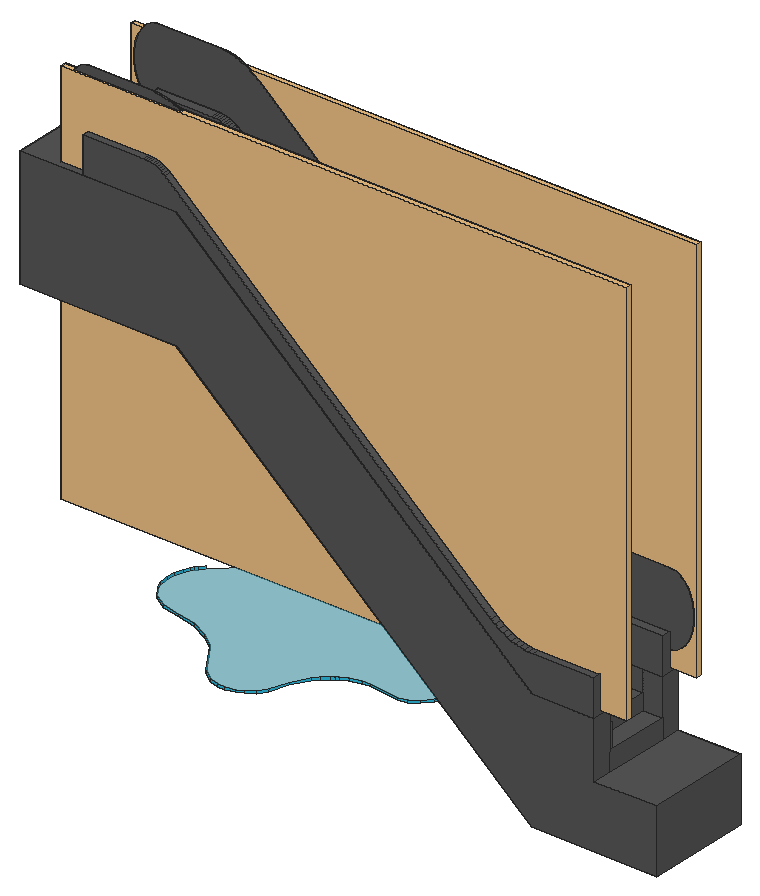
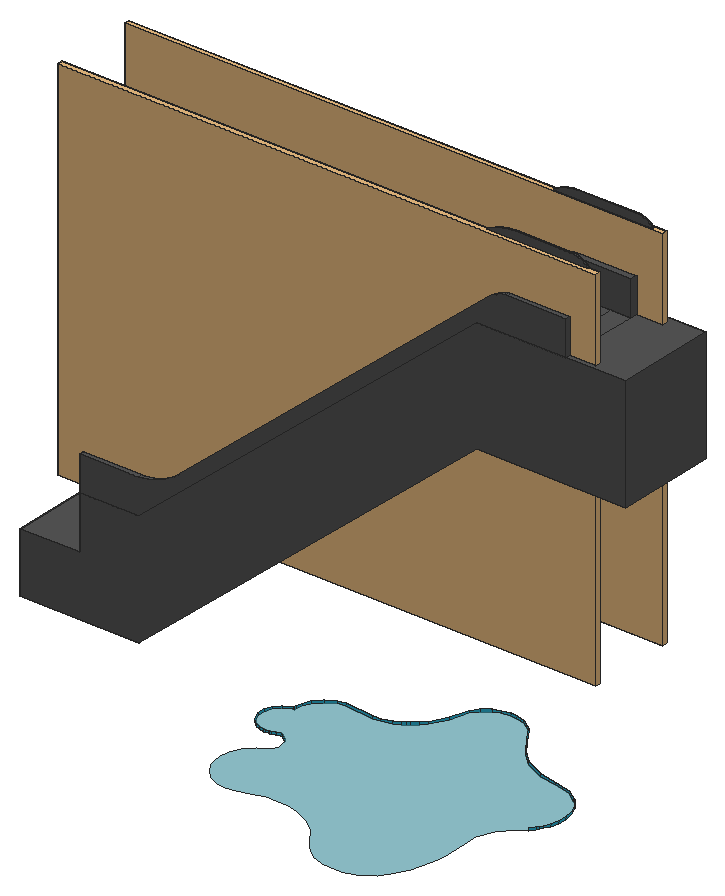
# SketchUp Ruby script. Lengths in inches.
U = 1.inch
M = Sketchup.active_model
def pt(a) = Geom::Point3d.new(a.map { |v| v * U })
def face(e, loops, mat)
  f = e.add_face(loops[0].map { |a| pt(a) })
  loops[1..].each { |l| e.add_face(l.map { |a| pt(a) }).erase! }
  f.material = f.back_material = mat if mat
  f
end
# faces: each face lists its corners as indices into pts; further lists are holes
def faces(e, pts, list, mat = nil) = list.each { |f| face(e, (f[0].is_a?(Array) ? f : [f]).map { |l| l.map { |i| pts[i] } }, mat) }
# xy, xz, yz: faces in a plane at the given z, y or x. An outline is a flat list of corners, or four numbers for a rectangle; further outlines are holes
def ring(l) = l.size == 4 ? [[l[0], l[1]], [l[2], l[1]], [l[2], l[3]], [l[0], l[3]]] : l.each_slice(2).to_a
def flat(e, list, mat, &to3) = list.each { |f| face(e, (f[0].is_a?(Array) ? f : [f]).map { |l| ring(l).map { |u, v| to3.(u, v) } }, mat) }
def xy(e, z, list, mat = nil) = flat(e, list, mat) { |x, y| [x, y, z] }
def xz(e, y, list, mat = nil) = flat(e, list, mat) { |x, z| [x, y, z] }
def yz(e, x, list, mat = nil) = flat(e, list, mat) { |y, z| [x, y, z] }
def lines(e, pts, list) = list.each { |a, b| e.add_line(pt(pts[a]), pt(pts[b])) }
# prism: a flat outline (further loops are holes) pulled along v
def prism(e, loops, v, mat = nil)
  f = face(e, loops, mat); d = Geom::Vector3d.new(v.map { |x| x * U })
  f.pushpull(f.normal.samedirection?(d) ? d.length : -d.length)
end
def box(e, o, s, mat = nil) = prism(e, [[o, [o[0] + s[0], o[1], o[2]], [o[0] + s[0], o[1] + s[1], o[2]], [o[0], o[1] + s[1], o[2]]]], [0, 0, s[2]], mat)
def at(x, y, z, deg = 0) = Geom::Transformation.translation(pt([x, y, z])) * Geom::Transformation.rotation(ORIGIN, Z_AXIS, deg.degrees)
def axes(o, x, y, z) = Geom::Transformation.new([*x, 0, *y, 0, *z, 0, *pt(o).to_a, 1])
def part(name) = M.definitions.add(name)
# library, detail: a bought-in or finely detailed component or shape, given as its bounding box
def library(name, o, s) = part(name).tap { |d| box(d.entities, o, s) }
def detail(e, o, s) = box(e.add_group.entities, o, s)
def put(e, d, t, mat = nil) = e.add_instance(d, t).tap { |i| i.material = mat if mat }
def group(e, t, mat = nil) = e.add_group.tap { |g| g.transformation = t; g.material = mat if mat }.entities
root = M.entities
M.materials.add("[Color M06]").color = [86, 86, 86]
M.materials.add("[Water Pool Light]").color = [62, 149, 166]
M.materials["[Water Pool Light]"].alpha = 0.6
M.materials.add("[Water Sparkling]").color = [45, 182, 216]
c1 = library("Group9\#2",[-51.57,-27.17,6.46],[325.75,3.15,149.29])
c2 = part("Group8\#1")
prism(c2.entities,[[[-38.42,-26,8.24],[-37.21,-26,8.08],[-35.98,-26,8.03],[-35.98,-26,14.02],[-0.59,-26,14.02],[3.6,-26,14.2],[7.75,-26,14.75],[11.84,-26,15.65],[15.84,-26,16.91],[19.71,-26,18.52],[23.43,-26,20.45],[211.27,-26,128.91],[213.125,-26,129.875],[215.06,-26,130.68],[217.06,-26,131.31],[219.1,-26,131.76],[221.18,-26,132.03],[223.27,-26,132.125],[258.59,-26,132.125],[258.59,-26,126.14],[259.81,-26,126.2],[261.02,-26,126.35],[262.22,-26,126.62],[263.38,-26,126.99],[264.51,-26,127.45],[265.6,-26,128.02],[266.63,-26,128.68],[267.6,-26,129.42],[268.5,-26,130.25],[269.33,-26,131.15],[270.07,-26,132.12],[270.73,-26,133.15],[271.29,-26,134.23],[271.76,-26,135.36],[272.125,-26,136.53],[272.39,-26,137.72],[272.55,-26,138.9375],[272.6,-26,140.16],[272.55,-26,141.38],[272.39,-26,142.59],[272.125,-26,143.79],[271.76,-26,144.95],[271.29,-26,146.08],[270.73,-26,147.17],[270.07,-26,148.2],[269.33,-26,149.17],[268.5,-26,150.07],[267.6,-26,150.89],[266.63,-26,151.64],[265.6,-26,152.3],[264.51,-26,152.86],[263.38,-26,153.33],[262.22,-26,153.7],[261.02,-26,153.96],[259.81,-26,154.12],[258.59,-26,154.17],[223.27,-26,154.17],[219.26,-26,154],[215.27,-26,153.47],[211.35,-26,152.6],[207.52,-26,151.4],[203.81,-26,149.86],[200.24,-26,148],[12.4,-26,39.54],[10.39,-26,38.5],[8.3,-26,37.63],[6.13,-26,36.95],[3.92,-26,36.46],[1.67,-26,36.16],[-0.59,-26,36.0625],[-35.98,-26,36.0625],[-37.21,-26,36.01],[-38.42,-26,35.85],[-39.61,-26,35.59],[-40.78,-26,35.22],[-41.91,-26,34.75],[-42.99,-26,34.19],[-44.02,-26,33.53],[-44.99,-26,32.78],[-45.89,-26,31.96],[-46.72,-26,31.06],[-47.47,-26,30.09],[-48.12,-26,29.06],[-48.6875,-26,27.97],[-49.15,-26,26.84],[-49.52,-26,25.67],[-49.79,-26,24.48],[-49.95,-26,23.27],[-50,-26,22.05],[-49.95,-26,20.83],[-49.79,-26,19.61],[-49.52,-26,18.42],[-49.15,-26,17.25],[-48.6875,-26,16.125],[-48.12,-26,15.04],[-47.47,-26,14.01],[-46.72,-26,13.04],[-45.89,-26,12.14],[-44.99,-26,11.3125],[-44.02,-26,10.57],[-42.99,-26,9.91],[-41.91,-26,9.34],[-40.78,-26,8.875],[-39.61,-26,8.51]]],[0,0.8125,0])
c3 = part("Group7\#1")
prism(c3.entities,[[[-35.98,-31.5,14.02],[-35.98,-31.5,0],[0,-31.5,0],[204.57,-31.5,118.11],[258.59,-31.5,118.11],[258.59,-31.5,132.125],[223.27,-31.5,132.125],[222.02,-31.5,132.09],[220.76,-31.5,131.99],[219.52,-31.5,131.83],[218.28,-31.5,131.6],[217.06,-31.5,131.31],[215.85,-31.5,130.95],[214.67,-31.5,130.53],[213.51,-31.5,130.05],[212.37,-31.5,129.51],[211.27,-31.5,128.91],[23.41,-31.5,20.45],[21.2,-31.5,19.25],[18.93,-31.5,18.16],[16.61,-31.5,17.2],[14.24,-31.5,16.36],[11.83,-31.5,15.65],[9.39,-31.5,15.0625],[6.92,-31.5,14.61],[4.43,-31.5,14.28],[1.92,-31.5,14.08],[-0.59,-31.5,14.02]]],[0,11.8125,0])
c4 = part("Group8\#2")
prism(c4.entities,[[[-38.42,-26,8.24],[-37.21,-26,8.08],[-35.98,-26,8.03],[-35.98,-26,14.02],[-0.59,-26,14.02],[3.6,-26,14.2],[7.75,-26,14.75],[11.84,-26,15.65],[15.84,-26,16.91],[19.71,-26,18.52],[23.43,-26,20.45],[211.27,-26,128.91],[213.125,-26,129.875],[215.06,-26,130.68],[217.06,-26,131.31],[219.1,-26,131.76],[221.18,-26,132.03],[223.27,-26,132.125],[258.59,-26,132.125],[258.59,-26,126.14],[259.81,-26,126.2],[261.02,-26,126.35],[262.22,-26,126.62],[263.38,-26,126.99],[264.51,-26,127.45],[265.6,-26,128.02],[266.63,-26,128.68],[267.6,-26,129.42],[268.5,-26,130.25],[269.33,-26,131.15],[270.07,-26,132.12],[270.73,-26,133.15],[271.29,-26,134.23],[271.76,-26,135.36],[272.125,-26,136.53],[272.39,-26,137.72],[272.55,-26,138.9375],[272.6,-26,140.16],[272.55,-26,141.38],[272.39,-26,142.59],[272.125,-26,143.79],[271.76,-26,144.95],[271.29,-26,146.08],[270.73,-26,147.17],[270.07,-26,148.2],[269.33,-26,149.17],[268.5,-26,150.07],[267.6,-26,150.89],[266.63,-26,151.64],[265.6,-26,152.3],[264.51,-26,152.86],[263.38,-26,153.33],[262.22,-26,153.7],[261.02,-26,153.96],[259.81,-26,154.12],[258.59,-26,154.17],[223.27,-26,154.17],[219.26,-26,154],[215.27,-26,153.47],[211.35,-26,152.6],[207.52,-26,151.4],[203.81,-26,149.86],[200.24,-26,148],[12.4,-26,39.54],[10.39,-26,38.5],[8.3,-26,37.63],[6.13,-26,36.95],[3.92,-26,36.46],[1.67,-26,36.16],[-0.59,-26,36.0625],[-35.98,-26,36.0625],[-37.21,-26,36.01],[-38.42,-26,35.85],[-39.61,-26,35.59],[-40.78,-26,35.22],[-41.91,-26,34.75],[-42.99,-26,34.19],[-44.02,-26,33.53],[-44.99,-26,32.78],[-45.89,-26,31.96],[-46.72,-26,31.06],[-47.47,-26,30.09],[-48.12,-26,29.06],[-48.6875,-26,27.97],[-49.15,-26,26.84],[-49.52,-26,25.67],[-49.79,-26,24.48],[-49.95,-26,23.27],[-50,-26,22.05],[-49.95,-26,20.83],[-49.79,-26,19.61],[-49.52,-26,18.42],[-49.15,-26,17.25],[-48.6875,-26,16.125],[-48.12,-26,15.04],[-47.47,-26,14.01],[-46.72,-26,13.04],[-45.89,-26,12.14],[-44.99,-26,11.3125],[-44.02,-26,10.57],[-42.99,-26,9.91],[-41.91,-26,9.34],[-40.78,-26,8.875],[-39.61,-26,8.51]]],[0,0.8125,0])
c5 = part("Group\#7")
put(c5.entities,c1,axes([389.09,-25,81.45],[-1.32087,0,0],[0,-1.27,0],[0,0,1.97633]))
g1 = group(c5.entities,at(0,0,0))
put(g1,c2,axes([389.09,40,90.88],[-1.32087,0,0],[0,-1.27,0],[0,0,1.97633]))
put(g1,c3,axes([389.09,40,90.88],[-1.32087,0,0],[0,-1.27,0],[0,0,1.97633]))
put(g1,c4,axes([389.09,-25,90.88],[-1.32087,0,0],[0,-1.27,0],[0,0,1.97633]))
g2 = group(g1,at(0,0,0))
xy(g2,0,[[389.09,0,484.2,80.01]])
xy(g2,48.01,[[436.62,0,484.2,80.01]])
xy(g2,62.63,[[422.02,15,436.62,65.01]])
xy(g2,74.76,[[399.75,15,422.02,65.01]])
xy(g2,83.13,[[377.47,15,399.75,65.01]])
xy(g2,90.88,[[389.09,0,436.62,15],[389.09,65.01,436.62,80.01]])
xy(g2,100.22,[[356.01,15,378.28,65.01]])
xy(g2,118.11,[[335.29,15,357.57,65.01]])
xy(g2,118.58,[[389.87,0,436.62,15]])
xy(g2,136.01,[[314.57,15,336.85,65.01]])
xy(g2,153.9,[[293.86,15,316.13,65.01]])
xy(g2,171.8,[[273.14,15,295.42,65.01]])
xy(g2,189.7,[[252.42,15,274.7,65.01]])
xy(g2,207.59,[[231.71,15,253.98,65.01]])
xy(g2,225.49,[[210.99,15,233.27,65.01]])
xy(g2,233.42,[[0,0,118.88,80.01]])
xy(g2,243.38,[[190.28,15,212.55,65.01]])
xy(g2,261.28,[[169.56,15,191.84,65.01]])
xy(g2,279.18,[[148.84,15,171.12,65.01]])
xy(g2,297.07,[[128.125,15,150.4,65.01]])
xy(g2,314.97,[[107.41,15,129.6875,65.01]])
xy(g2,324.3,[[0,0,47.53,0,47.53,65.01,118.88,65.01,118.88,80.01,0,80.01],[47.53,0,118.88,15],[47.53,15,63.67,65.01],[63.67,15,85.95,65.01],[85.95,15,108.22,65.01]])
xy(g2,352,[[47.53,0,94.18,15]])
xz(g2,0,[[389.09,0,484.2,0,484.2,48.01,436.62,48.01,436.62,90.88,389.09,90.88,118.88,324.3,0,324.3,0,233.42,118.88,233.42],[389.09,90.88,436.62,90.88,436.62,118.58,389.87,118.58,386.55,118.71,383.25,119.1,379.95,119.75,376.69,120.65,373.46,121.8125,370.28,123.22,367.15,124.88,364.09,126.78,361.09,128.92,358.18,131.29,110.04,345.65,108.58,346.83,107.08,347.9,105.54,348.85,103.98,349.68,102.39,350.39,100.77,350.97,99.14,351.42,97.49,351.74,95.84,351.9375,94.18,352,47.53,352,47.53,324.3,118.88,324.3]])
xz(g2,15,[[422.02,62.63,436.62,90.88],[399.75,74.76,422.02,90.88],[377.47,83.13,389.09,90.88],[389.09,83.13,399.75,90.88],[389.09,90.88,378.28,100.22,357.57,118.11,336.85,136.01,316.13,153.9,295.42,171.8,274.7,189.7,253.98,207.59,233.27,225.49,212.55,243.38,191.84,261.28,171.12,279.18,150.4,297.07,129.6875,314.97,118.88,324.3,47.53,324.3,47.53,352,94.18,352,95.84,351.9375,97.49,351.74,99.14,351.42,100.77,350.97,102.39,350.39,103.98,349.68,105.54,348.85,107.08,347.9,108.58,346.83,110.04,345.65,358.18,131.29,361.09,128.92,364.09,126.78,367.15,124.88,370.28,123.22,373.46,121.8125,376.69,120.65,379.95,119.75,383.25,119.1,386.55,118.71,389.87,118.58,436.62,118.58,436.62,90.88]])
xz(g2,65.01,[[422.02,62.63,436.62,90.88],[399.75,74.76,422.02,90.88],[377.47,83.13,389.09,90.88],[389.09,83.13,399.75,90.88]])
xz(g2,80.01,[[389.09,0,118.88,233.42,0,233.42,0,324.3,118.88,324.3,389.09,90.88,436.62,90.88,436.62,48.01,484.2,48.01,484.2,0]])
yz(g2,0,[[0,233.42,80.01,324.3]])
yz(g2,47.53,[[0,324.3,15,352]])
yz(g2,377.47,[[15,83.13,65.01,90.88]])
yz(g2,399.75,[[15,74.76,65.01,83.13]])
yz(g2,422.02,[[15,62.63,65.01,74.76]])
yz(g2,436.62,[[0,48.01,15,90.88],[15,48.01,65.01,62.63],[65.01,48.01,80.01,90.88],[0,90.88,15,118.58]])
yz(g2,484.2,[[0,0,80.01,48.01]])
p = [[389.09,80.01,0],[389.09,0,0],[118.88,0,233.42],[118.88,80.01,233.42],[378.28,15,100.22],[389.09,15,90.88],
  [389.09,0,90.88],[118.88,0,324.3],[118.88,15,324.3],[129.6875,15,314.97],[150.4,15,297.07],[171.12,15,279.18],
  [191.84,15,261.28],[212.55,15,243.38],[233.27,15,225.49],[253.98,15,207.59],[274.7,15,189.7],[295.42,15,171.8],
  [316.13,15,153.9],[336.85,15,136.01],[357.57,15,118.11],[378.28,65.01,100.22],[377.47,15,90.88],[377.47,65.01,90.88],
  [357.57,65.01,118.11],[356.01,15,100.22],[356.01,65.01,100.22],[336.85,65.01,136.01],[335.29,15,118.11],[335.29,65.01,118.11],
  [389.87,15,118.58],[386.55,15,118.71],[386.55,0,118.71],[389.87,0,118.58],[383.25,15,119.1],[383.25,0,119.1],
  [379.95,15,119.75],[379.95,0,119.75],[376.69,15,120.65],[376.69,0,120.65],[373.46,15,121.8125],[373.46,0,121.8125],
  [370.28,15,123.22],[370.28,0,123.22],[367.15,15,124.88],[367.15,0,124.88],[364.09,15,126.78],[364.09,0,126.78],
  [361.09,15,128.92],[361.09,0,128.92],[358.18,15,131.29],[358.18,0,131.29],[110.04,15,345.65],[110.04,0,345.65],
  [316.13,65.01,153.9],[314.57,15,136.01],[314.57,65.01,136.01],[295.42,65.01,171.8],[293.86,15,153.9],[293.86,65.01,153.9],
  [274.7,65.01,189.7],[273.14,15,171.8],[273.14,65.01,171.8],[253.98,65.01,207.59],[252.42,15,189.7],[252.42,65.01,189.7],
  [233.27,65.01,225.49],[231.71,15,207.59],[231.71,65.01,207.59],[212.55,65.01,243.38],[210.99,15,225.49],[210.99,65.01,225.49],
  [191.84,65.01,261.28],[190.28,15,243.38],[190.28,65.01,243.38],[171.12,65.01,279.18],[169.56,15,261.28],[169.56,65.01,261.28],
  [150.4,65.01,297.07],[148.84,15,279.18],[148.84,65.01,279.18],[129.6875,65.01,314.97],[128.125,15,297.07],[128.125,65.01,297.07],
  [108.22,65.01,324.3],[108.22,15,324.3],[107.41,15,314.97],[107.41,65.01,314.97],[108.58,15,346.83],[108.58,0,346.83],
  [107.08,15,347.9],[107.08,0,347.9],[105.54,15,348.85],[105.54,0,348.85],[103.98,15,349.68],[103.98,0,349.68],
  [102.39,15,350.39],[102.39,0,350.39],[100.77,15,350.97],[100.77,0,350.97],[99.14,15,351.42],[99.14,0,351.42],
  [97.49,15,351.74],[97.49,0,351.74],[95.84,15,351.9375],[95.84,0,351.9375],[94.18,15,352],[94.18,0,352]]
faces(g2,p,[[0,1,2,3],[4,5,6,7,8,9,10,11,12,13,14,15,16,17,18,19,20],[21,4,22,23],[24,20,25,26],[27,19,28,29],[30,31,32,33],[31,34,35,32],[34,36,37,35],
  [36,38,39,37],[38,40,41,39],[40,42,43,41],[42,44,45,43],[44,46,47,45],[46,48,49,47],[48,50,51,49],[50,52,53,51],
  [54,18,55,56],[57,17,58,59],[60,16,61,62],[63,15,64,65],[66,14,67,68],[69,13,70,71],[72,12,73,74],[75,11,76,77],
  [78,10,79,80],[81,9,82,83],[84,85,86,87],[52,88,89,53],[88,90,91,89],[90,92,93,91],[92,94,95,93],[94,96,97,95],
  [96,98,99,97],[98,100,101,99],[100,102,103,101],[102,104,105,103],[104,106,107,105]])
c6 = part("Group11\#1")
xz(c6.entities,-19.6875,[[-35.98,-19.69,-35.98,0,0,0,204.57,118.11,258.59,118.11,258.59,98.43,204.57,98.43,0,-19.69]])
xz(c6.entities,19.6875,[[-35.98,-19.69,0,-19.69,204.57,98.43,258.59,98.43,258.59,118.11,204.57,118.11,0,0,-35.98,0]])
p = [[0,-19.6875,0],[0,-31.5,0],[204.57,-31.5,118.11],[204.57,-19.6875,118.11],[0,19.6875,0],[0,31.5,0],
  [204.57,31.5,118.11],[204.57,19.6875,118.11]]
faces(c6.entities,p,[[0,1,2,3],[4,5,6,7]])
c7 = library("Group9\#1",[-51.57,-27.17,6.46],[325.75,3.15,149.29])
xy(root,20.71,[[285.14,260.64,292.29,262.02,297.26,264.26,303.02,268.7,307.42,274.49,311.91,288.48,318.44,300.88,322.16,305.12,326.4,308.8125,328.71,310.44,331.11,311.91,336.1875,314.34,344.3,316.67,349.9,317.29,373.49,314.65,379.82,316.19,386.78,320.36,392.01,326.58,394.54,332.57,395.35,337.39,395.4,339.02,396.5,339.28,402.51,342.3,406.89,347.41,408.79,352.69,408.67,359.41,405.28,366.47,402.8,368.82,402.01,369.57,400.11,370.52,399.9375,370.6,396.98,372.07,392.54,372.81,391.42,372.81,389.25,372.52,388.44,372.41,386.98,372.0625,384.87,371.26,380.99,370.3,379.15,370.78,374,375.26,372.99,381.41,375.49,386.45,378.01,388.36,383.44,391.84,389.86,399.08,393.09,406.125,394.39,413.77,394.03,419.58,391.81,427.01,387.73,433.6,382.09,438.92,375.26,442.59,372.94,443.3,371.35,443.56,365.78,444.49,358.06,443.74,349.18,440.48,345.72,439.32,342.2,438.39,338.62,437.7,335.01,437.24,320.48,437.85,313.41,439.59,300.27,445.8,297.28,447.88,291.74,452.62,282.8,464.08,278.17,470.42,274.42,474.08,267.96,478.54,263.21,480.75,258.21,482.3125,250.43,483.36,242.59,482.84,239.94,482.01,232.61,479.72,228.02,477.2,221.88,472.31,216.84,466.29,210.42,454.01,205.55,437.88,204.67,432.32,204.16,426.72,204.93,409.88,204.6,395.97,199.66,382.97,190.66,372.36,185.18,367.91,182.23,364.22,180.53,362.1,179.32,359.76,177.12,355.49,175.58,349.29,175.3,342.9,176.89,334.54,179.07,329.6875,179.51,328.71,180.37,327.58,183.38,323.65,184.68,321.95,185.875,321.17,195.29,314.93,207.75,312.44,222.15,309.47,237.2,302,246.85,293.88,256.8,280.34,263.78,269.07,272.69,262.85,279.6875,260.875]],"[Water Pool Light]")
xz(root,372.81,[[391.42,20.71,392.54,22.57]],"[Water Sparkling]")
p = [[279.6875,260.875,22.57],[285.14,260.64,22.57],[285.14,260.64,20.71],[279.6875,260.875,20.71],[292.29,262.02,22.57],[292.29,262.02,20.71],
  [272.69,262.85,22.57],[272.69,262.85,20.71],[297.26,264.26,22.57],[297.26,264.26,20.71],[263.78,269.07,22.57],[263.78,269.07,20.71],
  [303.02,268.7,22.57],[303.02,268.7,20.71],[307.42,274.49,22.57],[307.42,274.49,20.71],[256.8,280.34,22.57],[256.8,280.34,20.71],
  [311.91,288.48,22.57],[311.91,288.48,20.71],[246.85,293.88,22.57],[246.85,293.88,20.71],[318.44,300.88,22.57],[318.44,300.88,20.71],
  [237.2,302,22.57],[237.2,302,20.71],[322.16,305.12,22.57],[322.16,305.12,20.71],[222.15,309.47,22.57],[222.15,309.47,20.71],
  [326.4,308.8125,22.57],[326.4,308.8125,20.71],[328.71,310.44,22.57],[328.71,310.44,20.71],[207.75,312.44,22.57],[207.75,312.44,20.71],
  [331.11,311.91,22.57],[331.11,311.91,20.71],[336.1875,314.34,22.57],[336.1875,314.34,20.71],[195.29,314.93,22.57],[195.29,314.93,20.71],
  [344.3,316.67,22.57],[344.3,316.67,20.71],[349.9,317.29,22.57],[373.49,314.65,22.57],[373.49,314.65,20.71],[349.9,317.29,20.71],
  [379.82,316.19,22.57],[379.82,316.19,20.71],[185.875,321.17,22.57],[185.875,321.17,20.71],[386.78,320.36,22.57],[386.78,320.36,20.71],
  [392.01,326.58,22.57],[392.01,326.58,20.71],[184.68,321.95,22.57],[184.68,321.95,20.71],[183.38,323.65,22.57],[183.38,323.65,20.71],
  [180.37,327.58,22.57],[180.37,327.58,20.71],[394.54,332.57,22.57],[394.54,332.57,20.71],[179.51,328.71,22.57],[179.51,328.71,20.71],
  [179.07,329.6875,22.57],[179.07,329.6875,20.71],[176.89,334.54,22.57],[176.89,334.54,20.71],[395.35,337.39,22.57],[395.35,337.39,20.71],
  [175.3,342.9,22.57],[175.3,342.9,20.71],[395.4,339.02,22.57],[395.4,339.02,20.71],[396.5,339.28,22.57],[396.5,339.28,20.71],
  [402.51,342.3,22.57],[402.51,342.3,20.71],[406.89,347.41,22.57],[406.89,347.41,20.71],[175.58,349.29,22.57],[175.58,349.29,20.71],
  [408.79,352.69,22.57],[408.79,352.69,20.71],[177.12,355.49,22.57],[177.12,355.49,20.71],[408.67,359.41,22.57],[408.67,359.41,20.71],
  [179.32,359.76,22.57],[179.32,359.76,20.71],[405.28,366.47,22.57],[405.28,366.47,20.71],[180.53,362.1,22.57],[180.53,362.1,20.71],
  [182.23,364.22,22.57],[182.23,364.22,20.71],[185.18,367.91,22.57],[185.18,367.91,20.71],[402.8,368.82,22.57],[402.8,368.82,20.71],
  [402.01,369.57,22.57],[402.01,369.57,20.71],[400.11,370.52,22.57],[400.11,370.52,20.71],[380.99,370.3,22.57],[379.15,370.78,22.57],
  [379.15,370.78,20.71],[380.99,370.3,20.71],[384.87,371.26,22.57],[384.87,371.26,20.71],[399.9375,370.6,22.57],[399.9375,370.6,20.71],
  [396.98,372.07,22.57],[396.98,372.07,20.71],[374,375.26,22.57],[374,375.26,20.71],[386.98,372.0625,22.57],[386.98,372.0625,20.71],
  [388.44,372.41,22.57],[388.44,372.41,20.71],[392.54,372.81,22.57],[392.54,372.81,20.71],[389.25,372.52,22.57],[389.25,372.52,20.71],
  [391.42,372.81,22.57],[391.42,372.81,20.71]]
faces(root,p,[[0,1,2,3],[1,4,5,2],[6,0,3,7],[4,8,9,5],[10,6,7,11],[8,12,13,9],[12,14,15,13],[16,10,11,17],
  [14,18,19,15],[20,16,17,21],[18,22,23,19],[24,20,21,25],[22,26,27,23],[28,24,25,29],[26,30,31,27],[30,32,33,31],
  [34,28,29,35],[32,36,37,33],[36,38,39,37],[40,34,35,41],[38,42,43,39],[44,45,46,47],[45,48,49,46],[50,40,41,51],
  [48,52,53,49],[42,44,47,43],[52,54,55,53],[56,50,51,57],[58,56,57,59],[60,58,59,61],[54,62,63,55],[64,60,61,65],
  [66,64,65,67],[68,66,67,69],[62,70,71,63],[72,68,69,73],[70,74,75,71],[74,76,77,75],[76,78,79,77],[78,80,81,79],
  [82,72,73,83],[80,84,85,81],[86,82,83,87],[84,88,89,85],[90,86,87,91],[88,92,93,89],[94,90,91,95],[96,94,95,97],
  [98,96,97,99],[92,100,101,93],[100,102,103,101],[102,104,105,103],[106,107,108,109],[110,106,109,111],[104,112,113,105],[112,114,115,113],
  [107,116,117,108],[118,110,111,119],[120,118,119,121],[114,122,123,115],[124,120,121,125],[126,124,125,127]],"[Water Sparkling]")
g3 = group(root,at(139.1,248.43,17.43),"[Color M06]")
put(g3,c5,at(0,0,0))
put(g3,c6,axes([389.09,41.49,81.45],[-1.32087,0,0],[0,-1.27,0],[0,0,1.97633]))
put(g3,c7,axes([389.09,41.49,81.45],[-1.32087,0,0],[0,-1.27,0],[0,0,1.97633]))
